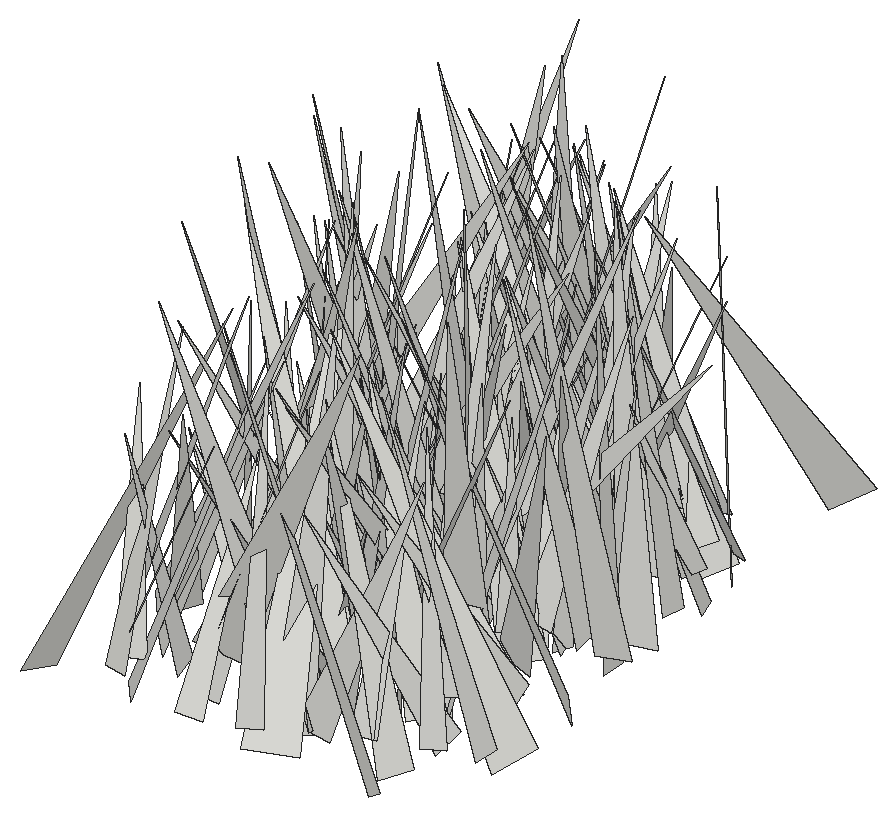
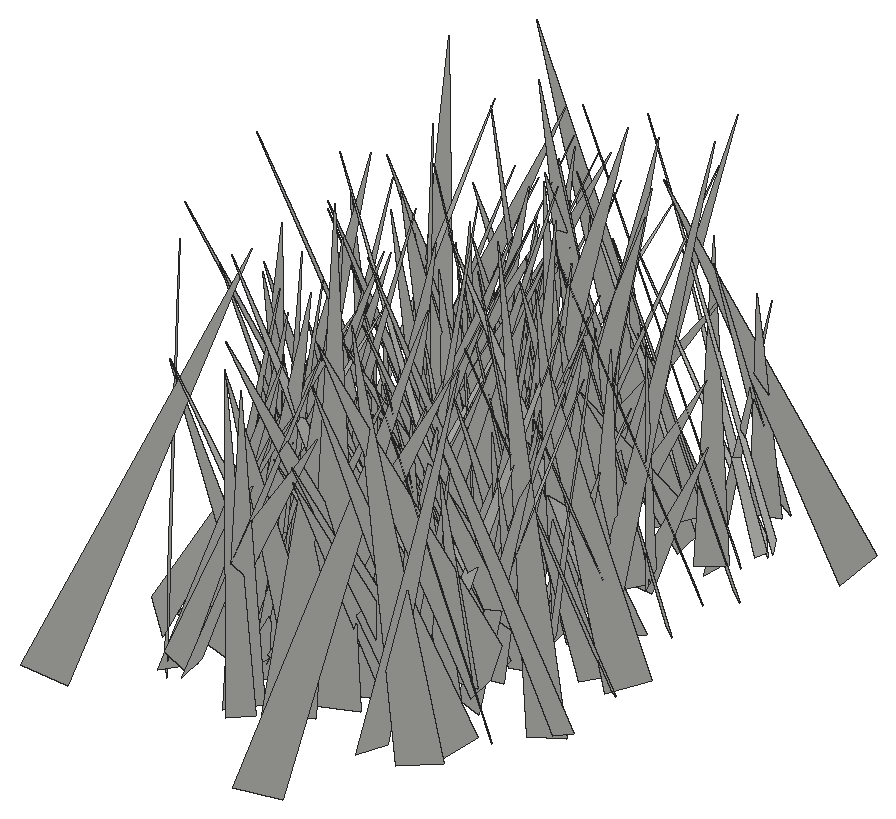
# SketchUp Ruby script. Lengths in inches.
U = 1.inch
M = Sketchup.active_model
def pt(a) = Geom::Point3d.new(a.map { |v| v * U })
def face(e, loops, mat)
  f = e.add_face(loops[0].map { |a| pt(a) })
  loops[1..].each { |l| e.add_face(l.map { |a| pt(a) }).erase! }
  f.material = f.back_material = mat if mat
  f
end
# faces: each face lists its corners as indices into pts; further lists are holes
def faces(e, pts, list, mat = nil) = list.each { |f| face(e, (f[0].is_a?(Array) ? f : [f]).map { |l| l.map { |i| pts[i] } }, mat) }
# xy, xz, yz: faces in a plane at the given z, y or x. An outline is a flat list of corners, or four numbers for a rectangle; further outlines are holes
def ring(l) = l.size == 4 ? [[l[0], l[1]], [l[2], l[1]], [l[2], l[3]], [l[0], l[3]]] : l.each_slice(2).to_a
def flat(e, list, mat, &to3) = list.each { |f| face(e, (f[0].is_a?(Array) ? f : [f]).map { |l| ring(l).map { |u, v| to3.(u, v) } }, mat) }
def xy(e, z, list, mat = nil) = flat(e, list, mat) { |x, y| [x, y, z] }
def xz(e, y, list, mat = nil) = flat(e, list, mat) { |x, z| [x, y, z] }
def yz(e, x, list, mat = nil) = flat(e, list, mat) { |y, z| [x, y, z] }
def lines(e, pts, list) = list.each { |a, b| e.add_line(pt(pts[a]), pt(pts[b])) }
# prism: a flat outline (further loops are holes) pulled along v
def prism(e, loops, v, mat = nil)
  f = face(e, loops, mat); d = Geom::Vector3d.new(v.map { |x| x * U })
  f.pushpull(f.normal.samedirection?(d) ? d.length : -d.length)
end
def box(e, o, s, mat = nil) = prism(e, [[o, [o[0] + s[0], o[1], o[2]], [o[0] + s[0], o[1] + s[1], o[2]], [o[0], o[1] + s[1], o[2]]]], [0, 0, s[2]], mat)
def at(x, y, z, deg = 0) = Geom::Transformation.translation(pt([x, y, z])) * Geom::Transformation.rotation(ORIGIN, Z_AXIS, deg.degrees)
def axes(o, x, y, z) = Geom::Transformation.new([*x, 0, *y, 0, *z, 0, *pt(o).to_a, 1])
def part(name) = M.definitions.add(name)
# library, detail: a bought-in or finely detailed component or shape, given as its bounding box
def library(name, o, s) = part(name).tap { |d| box(d.entities, o, s) }
def detail(e, o, s) = box(e.add_group.entities, o, s)
def put(e, d, t, mat = nil) = e.add_instance(d, t).tap { |i| i.material = mat if mat }
def group(e, t, mat = nil) = e.add_group.tap { |g| g.transformation = t; g.material = mat if mat }.entities
root = M.entities
c1 = part("fur_instance\#9")
p = [[0.8125,0,1.79],[0.67,-0.02,1.48],[0,-0.11,0],[0,0.11,0]]
faces(c1.entities,p,[[0,1,2,3]])
put(root,c1,axes([81.48,137.05,-28.22],[-7.1733,-2.93015,0.73361],[-2.97558,6.52972,-3.01478],[-0.51951,3.05896,7.13815]))
put(root,c1,axes([78.98,145.2,-27.1],[-6.42976,0.15301,2.02637],[0.5172,6.6259,1.14077],[1.96522,-1.24316,6.3296]))
put(root,c1,axes([77.69,134.6,-27.1],[2.30646,3.84948,0.31393],[3.83736,-2.32546,0.32205],[-0.43787,-0.10267,4.47599]))
put(root,c1,axes([75.62,125.64,-28.22],[7.28902,-0.71217,0.57332],[-0.83779,-7.04721,1.89755],[-0.36604,1.94818,7.07364]))
put(root,c1,axes([78.68,126.33,-27.1],[-1.71851,4.03919,1.0736],[4.16688,1.74577,0.10182],[0.32374,-1.02868,4.3884]))
put(root,c1,axes([78.98,131.57,-27.1],[3.80015,2.05854,2.10545],[1.83657,-4.34391,0.93228],[-2.30164,-0.0674,4.22014]))
put(root,c1,axes([80.16,130.65,-28.22],[-1.80359,3.13263,0.44398],[3.00697,1.53819,1.36218],[-0.98418,-1.04117,3.34825]))
put(root,c1,axes([77.28,131.38,-27.1],[4.12664,4.96749,0.53315],[4.97839,-4.14664,0.10195],[-0.41933,-0.34468,6.45715]))
put(root,c1,axes([78.79,125.42,-27.1],[1.97963,5.14738,0.61551],[5.06452,-2.06097,0.94673],[-1.10678,-0.22402,5.43306]))
put(root,c1,axes([78.51,134.91,-28.22],[-3.41876,-7.6362,0.72671],[-7.48826,3.49493,1.49637],[1.66304,0.03883,8.23167]))
put(root,c1,axes([76.58,135.68,-28.22],[5.22316,-4.20753,1.34718],[-4.41725,-5.01042,1.47756],[-0.07792,1.998,6.54228]))
put(root,c1,axes([78.89,136.52,-27.1],[-4.44854,-2.43941,1.67916],[-2.34276,4.75236,0.69742],[1.81157,0.15557,5.02532]))
put(root,c1,axes([76.66,142.34,-27.1],[4.45392,4.12687,0.87812],[4.21021,-4.26347,-1.31776],[0.27618,-1.55927,5.92722]))
put(root,c1,axes([79.07,128.49,-28.22],[-4.25466,-1.2014,1.34721],[-0.93808,4.41863,0.97784],[1.54219,-0.62673,4.31153]))
put(root,c1,axes([76.54,139.7,-28.22],[0.15208,-7.64456,1.76209],[-7.47072,0.39677,2.36609],[2.3943,1.72356,7.27077]))
put(root,c1,axes([76.94,136.1,-28.22],[3.93505,4.96293,0.50565],[4.97977,-3.8695,-0.7745],[0.29702,-0.87596,6.28613]))
put(root,c1,axes([79.64,139.68,-28.22],[-1.24841,-4.57565,0.91997],[-4.66472,1.19209,-0.401],[-0.15278,0.99186,4.72592]))
put(root,c1,axes([77.29,144.97,-27.1],[2.95876,-6.29379,1.88961],[-6.54545,-2.63888,1.45948],[0.58268,2.31543,6.79971]))
put(root,c1,axes([75.03,140.78,-27.1],[4.40787,6.56573,1.54887],[6.23945,-3.26461,-3.91775],[2.5646,-3.34225,6.86945]))
put(root,c1,axes([78.87,139.55,-27.1],[0.77798,-4.23548,0.16889],[-4.23878,-0.77834,0.00619],[-0.02442,0.16723,4.30633]))
put(root,c1,axes([80.6875,134.23,-28.22],[-2.26305,3.25436,0.20739],[3.19812,2.16563,0.91504],[-0.63708,-0.68879,3.8568]))
put(root,c1,axes([79.3,140.23,-27.1],[-0.34348,3.88251,1.09091],[4.02925,0.37671,-0.07204],[0.17064,-1.07988,3.89701]))
put(root,c1,axes([82.75,135.31,-28.22],[-7.866,-1.33504,0.19154],[-1.32695,7.45779,-2.51268],[-0.24134,2.50839,7.5725]))
put(root,c1,axes([78.52,133.16,-28.22],[-1.32926,4.80497,0.97182],[4.66035,1.55098,-1.29408],[1.52094,-0.553,4.81456]))
put(root,c1,axes([80.01,132.625,-28.22],[-1.55203,4.86816,1.43833],[5.0761,1.479,0.47157],[-0.03172,-1.51332,5.08777]))
put(root,c1,axes([78.07,129.77,-27.1],[4.2644,-2.86076,0.08373],[-2.8192,-4.22473,-0.76148],[-0.49304,-0.58632,5.07831]))
put(root,c1,axes([76.94,143.43,-27.1],[6.19791,-1.23637,0.25272],[-1.26158,-6.10069,1.0939],[-0.02993,1.12232,6.22464]))
put(root,c1,axes([80.3,133.85,-28.22],[-7.01527,0.64484,2.20419],[0.06996,7.14138,-1.86657],[2.29551,1.75305,6.79307]))
put(root,c1,axes([77.3,128.3,-27.1],[4.68379,1.41709,0.13919],[1.37897,-4.39495,-1.65779],[0.35492,-1.62533,4.60411]))
put(root,c1,axes([80.58,136.08,-28.22],[-4.6642,0.46344,0.8289],[0.1067,4.38406,-1.85075],[0.94364,1.79496,4.30631]))
put(root,c1,axes([80.23,140.91,-27.1],[-3.47678,-4.99975,0.07246],[-4.93171,3.44331,0.95532],[0.82523,-0.48669,6.01439]))
put(root,c1,axes([78.87,139.52,-27.1],[7.42059,-0.17453,3.00871],[-1.57677,-7.03899,3.48057],[-2.56838,3.81708,6.55601]))
put(root,c1,axes([79.76,142.23,-27.1],[-0.47471,-3.8388,0.84095],[-3.92781,0.49062,0.02236],[0.12592,0.83177,3.86797]))
put(root,c1,axes([77.48,129.24,-28.22],[4.35224,4.23695,0.82253],[4.28263,-4.09432,-1.57033],[0.53605,-1.68972,5.86752]))
put(root,c1,axes([77.29,127.63,-27.1],[6.01088,3.96881,0.98389],[4.08835,-5.80352,-1.56674],[0.06989,-1.84874,7.03046]))
put(root,c1,axes([79.42,133.3,-27.1],[-2.32023,4.26891,1.78267],[4.38145,2.66784,-0.68595],[1.48474,-1.20167,4.81004]))
put(root,c1,axes([77.77,132.2,-28.22],[4.67492,4.49227,1.13099],[4.6277,-4.45606,-1.42912],[0.20972,-1.8104,6.324]))
put(root,c1,axes([78.88,141.38,-28.22],[4.35751,-1.25814,0.68683],[-1.21703,-4.4086,-0.35441],[-0.75729,-0.15444,4.52164]))
put(root,c1,axes([81.03,134.83,-28.22],[-2.85386,-2.94003,0.13695],[-2.93623,2.85714,0.14971],[0.2028,-0.00613,4.09462]))
put(root,c1,axes([81.05,135.58,-28.22],[-7.46216,1.5868,2.36089],[1.65538,7.81249,-0.01867],[2.31332,-0.47194,7.62898]))
put(root,c1,axes([81.87,129.72,-27.1],[-2.56697,2.61634,0.35758],[2.51502,2.27032,1.44317],[-0.80484,-1.25014,3.36925]))
put(root,c1,axes([82.54,132.9,-27.1],[0.67019,6.07953,1.22269],[5.42193,-1.17133,2.85227],[-3.0097,-0.75637,5.41058]))
put(root,c1,axes([78.74,126.2,-28.22],[4.58247,4.01128,0.43645],[4.00699,-4.60163,0.22113],[-0.47421,-0.12046,6.08609]))
put(root,c1,axes([78.4375,138.42,-27.1],[1.11802,6.55656,0.88639],[6.4324,-0.86675,-1.70208],[1.54866,-1.13332,6.42972]))
put(root,c1,axes([80.76,127.33,-28.22],[-4.90566,2.32822,0.51514],[1.6552,4.17303,-3.098],[1.71648,2.62995,4.45965]))
put(root,c1,axes([77.71,135.98,-28.22],[0.54416,-5.67013,1.84078],[-5.27926,0.40028,2.79359],[2.76917,1.87733,4.9641]))
put(root,c1,axes([78.5625,134.27,-27.1],[6.55777,3.05775,0.67545],[3.00333,-6.58518,0.65252],[-0.88663,0.30968,7.20614]))
put(root,c1,axes([80.28,141.48,-27.1],[3.33409,-2.8819,1.80128],[-3.12207,-3.59416,0.02846],[-1.34262,1.20116,4.40689]))
put(root,c1,axes([81.86,134.37,-27.1],[-4.19914,-2.372,1.71601],[-2.90919,3.71707,-1.98087],[0.32817,2.60017,4.39719]))
put(root,c1,axes([80.34,132.8,-28.22],[-4.89725,-3.9807,3.26033],[-4.56553,5.43754,-0.21877],[2.37312,2.24631,6.30723]))
put(root,c1,axes([81.27,137.07,-27.1],[1.71301,-8.16044,0.92704],[-8.06805,-1.84913,-1.36891],[-1.53583,0.61199,8.22516]))
put(root,c1,axes([82.39,131.64,-27.1],[1.71463,6.79892,3.94816],[7.36353,-2.80488,1.63226],[-2.7553,-3.26505,6.81916]))
put(root,c1,axes([77.51,129.09,-27.1],[5.84897,4.9177,0.90335],[4.92852,-5.43629,-2.31659],[0.84231,-2.33947,7.282]))
put(root,c1,axes([81.66,133.66,-28.22],[4.59054,6.55576,1.84003],[6.00661,-4.94402,2.62946],[-3.20693,0.124,7.5589]))
put(root,c1,axes([81.26,147.92,-28.22],[6.1806,-4.85252,1.92283],[-3.89661,-6.27237,-3.30423],[-3.47285,-1.59827,7.12944]))
put(root,c1,axes([81.18,137.95,-28.22],[-3.91198,-5.41617,1.52932],[-5.50053,4.07361,0.35664],[1.19076,1.02376,6.67167]))
put(root,c1,axes([80.23,132.6,-28.22],[2.84043,2.51238,0.82611],[2.52394,-2.93724,0.2547],[-0.79009,-0.35083,3.78354]))
put(root,c1,axes([80.3,132.57,-28.22],[4.23217,0.79223,1.75299],[1.35483,-4.23497,-1.35698],[-1.36567,-1.74623,4.08626]))
put(root,c1,axes([81.36,138.15,-27.1],[4.43621,4.25023,1.48293],[3.65379,-4.61591,2.29927],[-2.62932,0.75659,5.69717]))
put(root,c1,axes([80.4375,140.71,-28.22],[5.48783,2.36239,1.1528],[1.72376,-5.24883,2.55038],[-1.98455,1.97355,5.40302]))
put(root,c1,axes([82.16,133.97,-28.22],[-6.61174,-0.50833,1.66504],[-0.62205,6.79727,-0.39495],[1.62598,0.53342,6.61948]))
put(root,c1,axes([81.83,140.83,-28.22],[-0.83956,4.61048,2.28414],[5.1209,0.52371,0.82514],[-0.50027,-2.37653,4.61309]))
put(root,c1,axes([81.19,141.36,-27.1],[-4.89219,1.92037,1.37183],[1.09822,4.64707,-2.5888],[2.08893,2.05431,4.57377]))
put(root,c1,axes([81.12,126.1,-28.22],[-0.73079,4.32054,0.1844],[4.30671,0.74406,-0.36572],[0.39156,-0.12013,4.36662]))
put(root,c1,axes([84.01,133.21,-27.1],[-6.46685,-0.99912,0.02995],[-0.985,6.33639,-1.3035],[-0.17003,1.29271,6.41243]))
put(root,c1,axes([79.41,134.83,-28.22],[3.43659,4.37627,1.35344],[4.55407,-3.08156,-1.59944],[0.49399,-2.03617,5.32951]))
put(root,c1,axes([82.32,129.17,-27.1],[-6.75805,0.02177,1.99006],[0.56326,6.77748,1.83863],[1.90881,-1.92284,6.50317]))
put(root,c1,axes([83.66,130.03,-27.1],[-6.02819,4.2729,0.70004],[4.32885,5.97346,0.81585],[0.09372,-1.07093,7.34378]))
put(root,c1,axes([82.58,133.3,-28.22],[-6.78403,-3.28205,0.63683],[-2.89291,6.48484,2.60352],[1.67585,-2.09175,7.07224]))
put(root,c1,axes([85.03,142.09,-28.22],[-5.71693,5.39586,0.3581],[5.20349,5.34707,2.50186],[-1.47216,-2.05434,7.45247]))
put(root,c1,axes([79.46,138.54,-27.1],[1.72384,-3.5656,0.8716],[-3.29525,-1.07913,2.10276],[1.61693,1.60212,3.35612]))
put(root,c1,axes([81.21,135,-28.22],[6.78257,3.66457,1.14232],[2.83952,-6.35069,3.51329],[-2.58286,2.6414,6.86216]))
put(root,c1,axes([79.28,132.61,-27.1],[6.86151,-4.43995,0.81428],[-4.49635,-6.85344,0.51929],[-0.39875,0.87961,8.15621]))
put(root,c1,axes([83.76,141.26,-27.1],[-3.5373,3.73043,1.14853],[3.88761,3.22863,1.48666],[-0.34887,-1.84596,4.92122]))
put(root,c1,axes([84.58,128.97,-27.1],[-2.08934,-4.39389,0.06996],[-3.98317,1.86084,-2.08523],[-1.85622,0.95264,4.39584]))
put(root,c1,axes([82.84,131.04,-27.1],[0.75585,6.87514,1.87347],[7.05211,-0.99202,0.79528],[-1.02238,-1.75986,6.87069]))
put(root,c1,axes([80.28,127.24,-28.22],[5.68273,3.19615,0.64935],[3.24559,-5.67036,-0.49352],[-0.32122,-0.74969,6.50117]))
put(root,c1,axes([83.65,137.85,-28.22],[-7.67624,-2.38765,2.18106],[-2.53698,7.93,-0.24775],[2.0054,0.89261,8.03519]))
put(root,c1,axes([79.25,142.21,-27.1],[6.564,-1.73993,0.0582],[-1.67851,-6.26496,2.01239],[0.46191,1.95953,6.48565]))
put(root,c1,axes([81.57,137.85,-27.1],[4.34106,2.99141,0.28027],[2.79242,-4.19877,1.56351],[-1.10882,1.13738,5.03476]))
put(root,c1,axes([82.95,133.75,-28.22],[-0.33834,3.74046,0.53618],[3.75079,0.26714,0.50319],[-0.45836,-0.57497,3.72187]))
put(root,c1,axes([81.53,143.91,-27.1],[2.47243,-7.62212,2.09201],[-7.90302,-2.41845,0.52868],[-0.12434,2.1542,7.99563]))
put(root,c1,axes([82.41,137.78,-28.22],[3.27584,-2.78093,0.2499],[-2.38988,-2.99185,-1.96583],[-1.44378,-1.35736,3.82103]))
put(root,c1,axes([81.06,134.82,-28.22],[3.86855,-0.79855,0.19754],[-0.81455,-3.85123,0.38332],[-0.11496,0.41562,3.93147]))
put(root,c1,axes([83.77,130.03,-27.1],[-3.58743,2.64736,0.43412],[2.66538,3.59954,0.07504],[0.30449,-0.3184,4.45786]))
put(root,c1,axes([82.12,142.71,-27.1],[3.81403,-1.87609,0.65313],[-1.66249,-3.78837,-1.17367],[-1.0874,-0.78844,4.08523]))
put(root,c1,axes([84.27,125.14,-27.1],[0.39127,5.5531,0.09038],[5.24022,-0.39914,1.8382],[-1.83989,0.04412,5.25462]))
put(root,c1,axes([80.85,140.17,-28.22],[2.35297,-5.60644,2.50548],[-6.03434,-1.6135,2.05656],[1.13856,3.03489,5.72182]))
put(root,c1,axes([84.61,128.04,-28.22],[-6.0397,-1.24718,1.08354],[-1.47294,5.92489,-1.39057],[0.74831,1.59618,6.00831]))
put(root,c1,axes([81.4,131.6,-28.22],[5.0608,-1.8582,0.79428],[-1.91101,-5.09708,0.2516],[-0.65714,0.51221,5.38529]))
put(root,c1,axes([81.67,139.78,-28.22],[4.40688,2.08061,0.00975],[2.02682,-4.29803,1.08102],[-0.47012,0.97349,4.75194]))
put(root,c1,axes([82.16,131.2,-27.1],[-2.28168,-4.43341,1.38047],[-4.1851,2.6298,1.52839],[2.0114,0.44265,4.74608]))
put(root,c1,axes([82.26,145.15,-27.1],[5.27875,-5.42072,0.96709],[-5.29735,-5.36505,-1.15714],[-1.50251,-0.12916,7.47733]))
put(root,c1,axes([85.59,142.29,-27.1],[-3.98273,-4.40716,0.90523],[-4.3967,3.55588,-2.0321],[-0.95477,2.0093,5.58174]))
put(root,c1,axes([84.37,137.43,-27.1],[-3.97928,1.73175,0.54979],[1.73454,4.01483,-0.09183],[0.54094,-0.13447,4.3388]))
put(root,c1,axes([85.59,134.45,-28.22],[-7.9003,-1.05971,0.99848],[-1.05239,7.96314,0.1246],[1.0062,0.00826,7.97008]))
put(root,c1,axes([84.47,125.91,-28.22],[-4.41357,6.91206,0.00056],[6.86097,4.38103,-0.99489],[0.83882,0.53496,8.14041]))
put(root,c1,axes([84.07,141.9,-28.22],[-3.76395,0.54517,1.33918],[0.93594,3.7652,1.09781],[1.1021,-1.33566,3.64133]))
put(root,c1,axes([83.07,140.05,-27.1],[4.24313,0.45781,1.20359],[0.34307,-4.39664,0.46288],[-1.24117,0.34981,4.24258]))
put(root,c1,axes([84.18,133.88,-27.1],[-4.88167,-3.98465,0.29136],[-3.56929,4.55624,2.50876],[1.79514,-1.77658,5.7805]))
put(root,c1,axes([81.06,137.38,-27.1],[7.00496,3.81978,0.96353],[3.93839,-6.83549,-1.53416],[-0.09034,-1.80938,7.82984]))
put(root,c1,axes([82.52,131.22,-28.22],[3.7872,-0.0255,0.26622],[0.02172,-3.73751,-0.66706],[-0.26655,-0.66693,3.72808]))
put(root,c1,axes([80.25,136.85,-27.1],[3.77376,6.10396,1.49671],[5.76595,-2.66802,-3.65722],[2.50047,-3.05991,6.17449]))
put(root,c1,axes([84.29,127.125,-28.22],[-5.70861,3.53079,2.01517],[3.32922,6.05385,-1.17592],[2.33318,0.00055,6.60847]))
put(root,c1,axes([82.75,132.95,-27.1],[4.81614,4.80746,1.57054],[5.00941,-4.83285,-0.56818],[-0.69571,-1.51836,6.78115]))
put(root,c1,axes([84.44,132.23,-28.22],[0.53786,-3.60504,0.14249],[-3.55289,-0.5543,-0.6129],[-0.62738,0.04841,3.59304]))
put(root,c1,axes([85.1,141.6,-27.1],[-7.14717,-1.7401,1.8273],[-1.33254,7.26397,1.70532],[2.14274,-1.28679,7.15555]))
put(root,c1,axes([86.23,137.26,-27.1],[-6.15592,-2.89241,0.11132],[-2.84807,6.09927,0.98037],[0.51666,-0.84058,6.73054]))
put(root,c1,axes([84.8,137.53,-27.1],[-5.4201,3.31702,1.28358],[3.06796,5.54385,-1.37151],[1.7994,0.53923,6.20476]))
put(root,c1,axes([82.44,141.18,-28.22],[5.43533,-0.93824,0.08866],[-0.80913,-4.91198,-2.3767],[-0.48317,-2.32876,4.97739]))
put(root,c1,axes([80.59,128.27,-27.1],[3.82613,-7.13137,0.63835],[-6.75778,-3.35774,2.99351],[2.36564,1.94225,7.51895]))
put(root,c1,axes([83.41,138.98,-27.1],[6.6915,4.26773,1.20587],[3.94044,-6.72308,1.92792],[-2.03484,1.01512,7.69888]))
put(root,c1,axes([83.98,135.33,-27.1],[1.01663,5.56132,0.68679],[5.60282,-1.02017,-0.03274],[-0.09106,-0.68151,5.65338]))
put(root,c1,axes([86.35,135.52,-27.1],[-1.63613,-6.00923,1.56488],[-6.02721,1.14742,-1.89548],[-1.49415,1.95172,5.93253]))
put(root,c1,axes([86.01,134.61,-27.1],[-6.75502,-2.37628,0.59319],[-2.11002,6.52988,2.13012],[1.24354,-1.82836,6.83664]))
put(root,c1,axes([84.92,132.91,-27.1],[1.57492,-4.967,1.49516],[-5.0252,-1.8484,-0.84719],[-1.28605,1.13987,5.14138]))
put(root,c1,axes([86.47,144.65,-27.1],[-6.23663,-1.3966,0.55844],[-1.37103,6.25805,0.33911],[0.61857,-0.21031,6.38209]))
put(root,c1,axes([87.96,142.54,-27.1],[-2.08516,6.03207,0.25096],[5.29839,1.7011,3.1353],[-2.89412,-1.23172,5.5591]))
put(root,c1,axes([88.58,125.85,-28.22],[-6.97142,-3.26118,0.0354],[-2.96258,6.29742,-3.28677],[-1.3637,2.99072,6.9594]))
put(root,c1,axes([84.95,144,-28.22],[3.99343,-3.31881,2.86458],[-3.84361,-4.5142,0.12826],[-2.10878,1.94301,5.19091]))
put(root,c1,axes([84.3,141.92,-27.1],[-1.65909,5.33475,1.21269],[5.33342,1.85943,-0.88312],[1.21852,-0.87506,5.51654]))
put(root,c1,axes([84.16,139.64,-27.1],[3.26385,-1.40609,1.47007],[-1.85279,-3.20219,1.05074],[-0.83985,1.59994,3.39496]))
put(root,c1,axes([82.42,136.68,-28.22],[6.6655,-1.52718,0.22941],[-1.49066,-6.62814,-0.81212],[-0.40351,-0.74118,6.78982]))
put(root,c1,axes([85.8,142.125,-28.22],[-6.8866,-1.44069,2.04712],[-1.4724,7.17733,0.09795],[2.02444,0.3193,7.035]))
put(root,c1,axes([85.1875,137.28,-28.22],[-3.08367,2.72536,1.78242],[3.08151,3.23588,0.38343],[1.05304,-1.48834,4.09751]))
put(root,c1,axes([86.23,143.42,-27.1],[-1.07248,-7.00957,0.36815],[-6.96342,1.01561,-0.94825],[-0.88342,0.50425,7.02746]))
put(root,c1,axes([87.12,133.3125,-27.1],[-4.6266,-2.97065,0.07987],[-2.96143,4.59663,-0.58091],[-0.24706,0.53178,5.46742]))
put(root,c1,axes([85.47,131.16,-27.1],[-2.10468,-4.52268,1.53831],[-4.75533,2.14388,-0.20306],[0.45584,1.48319,4.98428]))
put(root,c1,axes([86.59,141.73,-28.22],[-1.73257,6.85044,2.42635],[7.20837,1.30251,1.46979],[-0.92468,-2.68187,6.91158]))
put(root,c1,axes([83.5,134.92,-27.1],[4.06757,1.21437,0.51699],[1.31683,-3.847,-1.32426],[-0.08902,-1.4188,4.03313]))
put(root,c1,axes([83.39,146.09,-27.1],[5.22724,-1.35677,0.09683],[-1.28473,-5.05093,-1.4184],[-0.44684,-1.34966,5.21086]))
put(root,c1,axes([84.55,130.99,-27.1],[5.34642,-2.10558,1.0321],[-1.67954,-5.23165,-1.97278],[-1.63641,-1.50973,5.39684]))
put(root,c1,axes([84.77,132.78,-28.22],[4.36466,2.86173,1.95624],[3.18404,-4.55325,-0.44325],[-1.3705,-1.46462,5.20032]))
put(root,c1,axes([86.97,135.12,-28.22],[-5.2406,4.407,1.34408],[4.57378,5.22157,0.71269],[0.55566,-1.41624,6.81011]))
put(root,c1,axes([89.25,141.25,-28.22],[-7.14593,-4.06809,0.00282],[-3.91681,6.87864,-2.22635],[-1.09909,1.93614,7.91562]))
put(root,c1,axes([85.74,139.27,-28.22],[-0.63245,-3.70623,0.66325],[-3.76509,0.62047,-0.12308],[-0.01169,0.67448,3.75779]))
put(root,c1,axes([88.13,132.2,-27.1],[-6.75441,-2.93713,0.31923],[-2.94167,6.75982,-0.04619],[0.27431,0.1697,7.36523]))
put(root,c1,axes([86.68,142.78,-27.1],[0.19192,-5.71021,2.24229],[-6.02696,-0.59408,-0.99702],[-1.14462,2.17066,5.62577]))
put(root,c1,axes([84.37,129.66,-28.22],[-2.78435,-5.66723,3.39056],[-5.97834,3.72634,1.319],[2.80584,2.3158,6.17497]))
put(root,c1,axes([87.12,144.64,-27.1],[-0.99125,-4.30354,0.98962],[-4.28593,0.69339,-1.27766],[-1.06332,1.21702,4.22737]))
put(root,c1,axes([86.78,138.85,-27.1],[-3.90024,1.94852,0.94584],[2.05782,3.9414,0.36592],[0.67579,-0.75618,4.3445]))
put(root,c1,axes([86.33,143,-27.1],[-4.22717,-2.44585,1.01456],[-2.28976,4.33627,0.91336],[1.32985,-0.3083,4.79759]))
put(root,c1,axes([89.28,142.82,-27.1],[-4.75874,-5.64309,0.42264],[-5.39038,4.3522,-2.58279],[-1.72245,1.97043,6.91515]))
put(root,c1,axes([86.12,141.1,-27.1],[3.3067,2.95122,2.18217],[3.23124,-3.73382,0.15332],[-1.74087,-1.32466,4.4295]))
put(root,c1,axes([88.12,143.28,-28.22],[-6.01632,2.22797,0.81671],[2.32649,5.97644,0.83455],[0.46722,-1.07014,6.36109]))
put(root,c1,axes([87.125,139.59,-27.1],[-0.56263,-5.96411,0.83016],[-5.9756,0.45013,-0.816],[-0.74291,0.89616,5.93475]))
put(root,c1,axes([87.91,132.9,-28.22],[2.18391,-6.70079,0.42323],[-6.08063,-2.16263,-2.86325],[-2.84706,-0.52116,6.43986]))
put(root,c1,axes([84.54,140.8,-28.22],[5.42276,2.60915,0.23648],[2.58182,-5.41452,0.53583],[-0.44475,0.3811,5.9939]))
put(root,c1,axes([88.9,131.75,-27.1],[-5.72955,1.74546,0.28048],[1.75274,5.48455,1.67353],[-0.23061,-1.68113,5.75097]))
put(root,c1,axes([87.22,132.45,-28.22],[-6.98093,-2.98191,2.95578],[-3.56155,7.24267,-1.10492],[2.22346,2.23913,7.51028]))
put(root,c1,axes([88.3125,127.22,-28.22],[-5.80582,1.67481,0.45332],[1.66732,5.82342,-0.1609],[0.48013,0.02943,6.04042]))
put(root,c1,axes([87.42,136.62,-28.22],[-3.47043,-1.20582,0.35373],[-1.16309,3.47557,0.43669],[0.47575,-0.29913,3.64791]))
put(root,c1,axes([86.3125,129.92,-28.22],[2.87799,2.64757,1.74089],[2.94858,-3.09885,-0.16173],[-1.16026,-1.30792,3.90721]))
put(root,c1,axes([85.82,133.96,-27.1],[2.40691,-4.24835,1.2679],[-4.42272,-2.4014,0.34948],[-0.30924,1.27831,4.87028]))
put(root,c1,axes([88.05,129.05,-27.1],[-4.17135,3.80631,1.04328],[3.93898,4.10999,0.75433],[0.24669,-1.26356,5.59635]))
put(root,c1,axes([86.77,135.8,-28.22],[-1.60634,4.05647,0.77587],[4.09581,1.67158,-0.25963],[0.53033,-0.623,4.35521]))
put(root,c1,axes([87.53,130.28,-27.1],[-6.45449,2.84921,1.13675],[2.42101,6.35763,-2.18855],[1.88385,1.59157,6.70736]))
put(root,c1,axes([87.18,130.54,-28.22],[-4.49774,2.41965,1.22715],[2.26445,4.65664,-0.88215],[1.49428,0.22634,5.03052]))
put(root,c1,axes([84.69,127.69,-28.22],[2.29321,-4.71361,1.70331],[-4.8602,-1.63403,2.02152],[1.22385,2.34308,4.83635]))
put(root,c1,axes([86.75,134.71,-27.1],[-1.48065,3.15767,1.46809],[3.42197,1.61497,-0.02236],[0.64523,-1.31889,3.48751]))
put(root,c1,axes([87.33,126.875,-27.1],[0.66443,5.27954,0.01832],[5.19176,-0.65673,0.9642],[-0.95891,0.10252,5.2331]))
put(root,c1,axes([86.65,138.27,-28.22],[-5.03968,3.97301,2.20808],[3.85689,5.48236,-1.06156],[2.40517,-0.46656,6.329]))
put(root,c1,axes([85.33,138.6,-27.1],[3.14685,5.37097,0.90824],[5.43729,-3.03382,-0.89816],[0.32882,-1.23429,6.15981]))
put(root,c1,axes([87.41,136.53,-28.22],[-3.90689,0.46662,1.17538],[0.26281,4.03296,-0.72751],[1.23701,0.61693,3.86682]))
put(root,c1,axes([85,142.65,-27.1],[4.99939,-0.31235,0.02616],[-0.31267,-4.999,0.06629],[-0.02197,0.06779,5.0087]))
put(root,c1,axes([88.36,129.75,-28.22],[-4.86866,0.51762,1.11395],[0.97098,4.41082,2.19421],[0.75234,-2.34296,4.3769]))
put(root,c1,axes([85.25,134.07,-27.1],[4.54632,6.46757,0.61256],[6.48609,-4.47646,-0.87508],[0.36794,-1.0028,7.85702]))
put(root,c1,axes([85.17,129.85,-28.22],[6.47298,0.85818,0.33872],[0.84258,-6.4766,0.30739],[-0.37587,0.26066,6.52238]))
put(root,c1,axes([86.01,138.7,-27.1],[5.48383,-1.63022,0.30334],[-1.45467,-5.23263,-1.82362],[-0.79597,-1.66854,5.42259]))
put(root,c1,axes([90.64,130.14,-28.22],[-7.28796,2.50197,0.93453],[2.66483,6.99355,2.0583],[0.17855,-2.25345,7.42547]))
put(root,c1,axes([88.87,136.01,-27.1],[-6.26748,-0.84521,1.62615],[-0.68504,6.45447,0.7145],[1.69984,-0.51518,6.28372]))
put(root,c1,axes([89.85,138.86,-27.1],[-6.30755,-1.0303,0.95825],[-1.23667,6.15876,-1.51833],[0.67114,1.66527,6.20817]))
put(root,c1,axes([87.1,131.02,-28.22],[4.30738,5.01035,0.65824],[4.94004,-4.35705,0.83813],[-1.06435,0.05398,6.55397]))
put(root,c1,axes([82.84,137.67,-28.22],[5.03462,6.0848,0.40692],[5.07887,-3.8915,-4.64748],[3.37572,-3.22012,6.38538]))
put(root,c1,axes([87,135.67,-27.1],[0.12132,5.40428,1.16344],[5.42728,0.10479,-1.05269],[1.05091,-1.16504,5.30215]))
put(root,c1,axes([89.04,138.09,-28.22],[-0.74799,6.94474,2.29097],[7.27165,0.46217,0.97314],[-0.77532,-2.36525,6.91678]))
put(root,c1,axes([87.87,138.08,-27.1],[1.06055,3.50039,1.15885],[3.68372,-1.05849,-0.17402],[-0.16095,-1.16074,3.65339]))
put(root,c1,axes([87.25,132.1,-27.1],[5.45655,-4.97036,1.37233],[-4.9464,-5.60993,-0.6508],[-1.45634,0.43117,7.35221]))
put(root,c1,axes([89.36,136.53,-28.22],[-6.31895,-1.30533,1.91515],[-1.71826,6.37081,-1.32708],[1.5554,1.73484,6.31441]))
put(root,c1,axes([89.48,127.61,-27.1],[-0.14147,5.00237,0.6936],[4.87308,-0.04695,1.33257],[-1.32587,-0.70632,4.82369]))
put(root,c1,axes([89.54,131.72,-27.1],[-5.28354,-0.86585,0.73138],[-0.45173,4.80676,2.42722],[1.0395,-2.31209,4.77222]))
put(root,c1,axes([89.96,133.6875,-28.22],[-5.65228,-5.31186,0.60473],[-5.29476,5.68375,0.43618],[0.73959,0.09466,7.74428]))
put(root,c1,axes([90.21,135.48,-27.1],[-1.59145,-6.67923,2.98055],[-7.18236,0.85085,-1.92829],[-1.38185,3.26993,6.58988]))
put(root,c1,axes([88.83,141.18,-27.1],[2.63547,-2.52355,0.88422],[-2.24578,-2.7628,-1.19134],[-1.45143,-0.30736,3.44888]))
put(root,c1,axes([89.71,147.8,-27.1],[4.2838,-6.03866,0.74714],[-5.20831,-4.11147,-3.36808],[-3.14598,-1.41597,6.59337]))
put(root,c1,axes([88.38,143.52,-28.22],[-4.90081,-4.60842,2.76686],[-4.75517,5.4628,0.67611],[2.50627,1.35324,6.69315]))
put(root,c1,axes([86.8,134.9,-28.22],[0.27487,-5.90315,0.86813],[-5.62576,0.03312,2.00651],[1.98787,0.91,5.55848]))
put(root,c1,axes([90.98,128.32,-27.1],[-5.83458,-0.97839,0.23219],[-1.00024,5.78729,-0.74851],[0.10327,0.77686,5.8685]))
